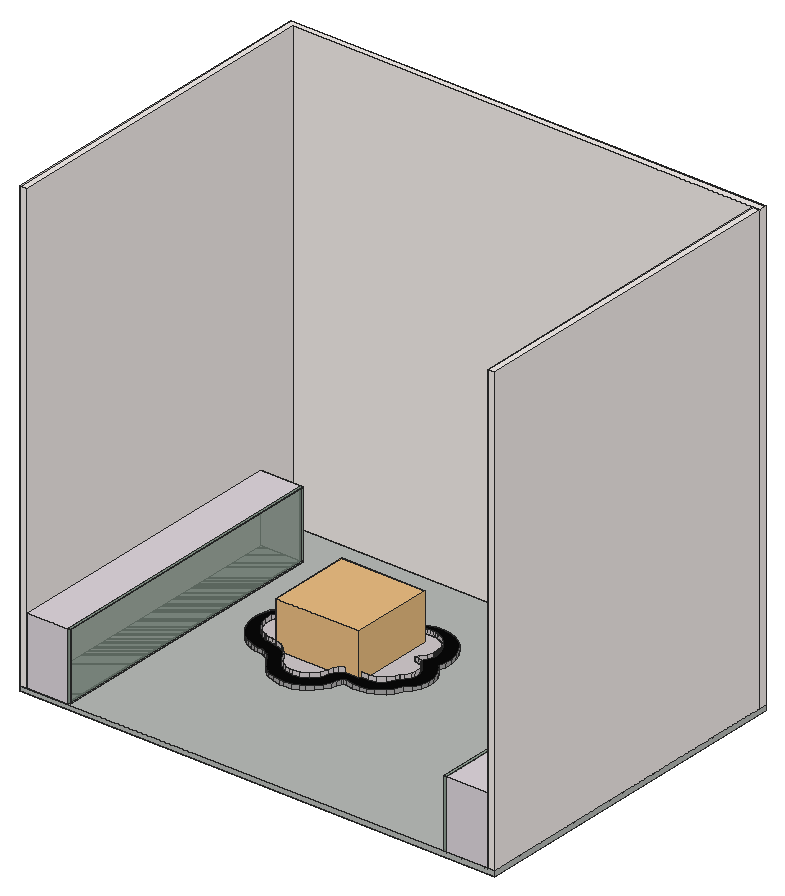
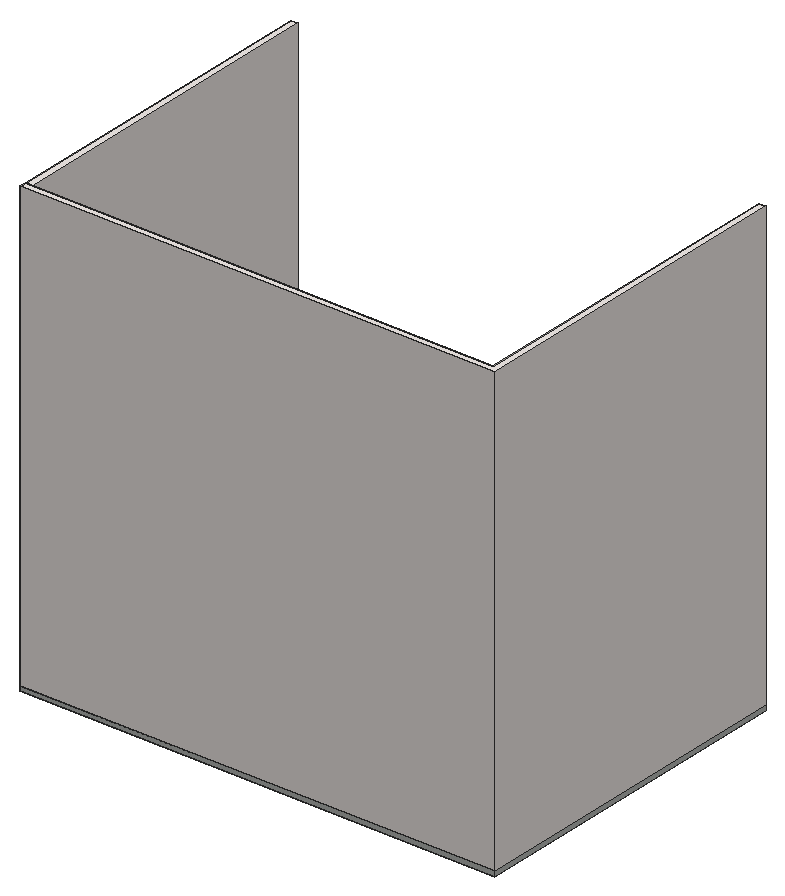
# SketchUp Ruby script. Lengths in inches.
U = 1.inch
M = Sketchup.active_model
def pt(a) = Geom::Point3d.new(a.map { |v| v * U })
def face(e, loops, mat)
  f = e.add_face(loops[0].map { |a| pt(a) })
  loops[1..].each { |l| e.add_face(l.map { |a| pt(a) }).erase! }
  f.material = f.back_material = mat if mat
  f
end
# faces: each face lists its corners as indices into pts; further lists are holes
def faces(e, pts, list, mat = nil) = list.each { |f| face(e, (f[0].is_a?(Array) ? f : [f]).map { |l| l.map { |i| pts[i] } }, mat) }
# xy, xz, yz: faces in a plane at the given z, y or x. An outline is a flat list of corners, or four numbers for a rectangle; further outlines are holes
def ring(l) = l.size == 4 ? [[l[0], l[1]], [l[2], l[1]], [l[2], l[3]], [l[0], l[3]]] : l.each_slice(2).to_a
def flat(e, list, mat, &to3) = list.each { |f| face(e, (f[0].is_a?(Array) ? f : [f]).map { |l| ring(l).map { |u, v| to3.(u, v) } }, mat) }
def xy(e, z, list, mat = nil) = flat(e, list, mat) { |x, y| [x, y, z] }
def xz(e, y, list, mat = nil) = flat(e, list, mat) { |x, z| [x, y, z] }
def yz(e, x, list, mat = nil) = flat(e, list, mat) { |y, z| [x, y, z] }
def lines(e, pts, list) = list.each { |a, b| e.add_line(pt(pts[a]), pt(pts[b])) }
# prism: a flat outline (further loops are holes) pulled along v
def prism(e, loops, v, mat = nil)
  f = face(e, loops, mat); d = Geom::Vector3d.new(v.map { |x| x * U })
  f.pushpull(f.normal.samedirection?(d) ? d.length : -d.length)
end
def box(e, o, s, mat = nil) = prism(e, [[o, [o[0] + s[0], o[1], o[2]], [o[0] + s[0], o[1] + s[1], o[2]], [o[0], o[1] + s[1], o[2]]]], [0, 0, s[2]], mat)
def at(x, y, z, deg = 0) = Geom::Transformation.translation(pt([x, y, z])) * Geom::Transformation.rotation(ORIGIN, Z_AXIS, deg.degrees)
def axes(o, x, y, z) = Geom::Transformation.new([*x, 0, *y, 0, *z, 0, *pt(o).to_a, 1])
def part(name) = M.definitions.add(name)
# library, detail: a bought-in or finely detailed component or shape, given as its bounding box
def library(name, o, s) = part(name).tap { |d| box(d.entities, o, s) }
def detail(e, o, s) = box(e.add_group.entities, o, s)
def put(e, d, t, mat = nil) = e.add_instance(d, t).tap { |i| i.material = mat if mat }
def group(e, t, mat = nil) = e.add_group.tap { |g| g.transformation = t; g.material = mat if mat }.entities
root = M.entities
M.materials.add("0209 AP 9428 SKY PINK").color = [243, 236, 233]
M.materials.add("0265 AP 7147 LAVENDER LAUGH").color = [222, 214, 220]
M.materials.add("Bricks_Tiles_D02_50cm").color = [9, 9, 9]
M.materials.add("Epoch Sky_ Double Herringbone (VR1MIV)").color = [184, 188, 184]
M.materials.add("[Stone_Granite_Midnite]").color = [209, 202, 204]
M.materials.add("[Stone_Vein_Gray]").color = [166, 165, 165]
M.materials.add("[Translucent Glass Corrugated]").color = [141, 158, 145]
M.materials["[Translucent Glass Corrugated]"].alpha = 0.8
c1 = part("Group\#1")
box(c1.entities,[0,0,0],[840,600,8])
c2 = library("Group\#44",[13.4,13.93,0],[164.31,164.31,140.86])
c3 = part("Group41\#1")
p = [[514.8125,1.1875,0],[1.1875,1.1875,0],[1.1875,118.8125,0],[514.8125,118.8125,0]]
lines(c3.entities,p,[[0,1],[1,2],[2,3],[3,0]])
c4 = part("Group42\#1")
xy(c4.entities,2.9375,[[1.1875,1.1875,514.8125,118.8125]])
c5 = part("Group40\#1")
prism(c5.entities,[[[516,120,0],[516,0,0],[0,0,0],[0,120,0]],[[1.1875,118.8125,0],[1.1875,1.1875,0],[514.8125,1.1875,0],[514.8125,118.8125,0]]],[0,0,5.875])
put(c5.entities,c3,at(0,0,0))
put(c5.entities,c4,at(0,0,0))
c6 = part("Group\#11")
xy(c6.entities,0,[[0,72,72,588]])
xy(c6.entities,120,[[0,72,72,588]])
xz(c6.entities,72,[[0,0,72,120]])
xz(c6.entities,588,[[0,0,72,120]])
yz(c6.entities,0,[[72,0,588,120]])
put(c6.entities,c5,axes([72,72,0],[0,1,0],[0,0,1],[1,0,0]),"[Translucent Glass Corrugated]")
xy(root,8,[[286.38,226.11,278.14,226.18,265.97,228.35,254.48,232.88,247.41,237.13,238.03,245.17,230.42,254.91,225.67,263.83,222.52,268.43,218.51,272.29,213.8,275.26,210.37,276.6875,204.93,277.92,198.67,278.46,192.125,279.62,185.71,281.35,177.5,284.68,171.69,287.91,166.19,291.64,162.76,294.44,159.52,297.46,151.1,307.73,146.6875,315.41,142.08,327.86,140.02,340.98,140.12,349.84,142.46,362.91,145.4375,371.25,151.91,382.84,160.55,392.92,168.89,400.18,170.02,404.39,169.07,412.74,168.71,420.7,170.62,441.81,170.86,444.46,171.88,448.31,173.58,454.71,174.94,459.85,181.06,474.55,193.58,493.52,208.59,506.3,231.23,515.95,240.97,517.6,260.68,516.94,265.53,515.95,274.96,513.01,291.39,503.95,296.1,500.41,299.76,497.09,306.35,489.73,313.41,479.34,318.33,474.84,325.77,471.91,332.44,471.86,337.55,473.39,353.76,478.27,366.45,479.05,379.05,477.32,391.06,473.13,402,466.67,411.46,458.18,421.13,444.28,425.8,432.45,428.06,419.94,427.81,407.23,425.05,394.82,432.1,387.375,438.96,375.57,442.49,362.39,442.79,352.14,440.05,338.77,433.89,326.58,424.77,316.43,419.17,306,411.6,296.89,398.99,287.43,388.13,282.72,376.55,280.26,364.72,280.16,350.18,282.69,346.97,281.54,344.64,279.05,342.91,272.72,340.36,264.88,334.63,253.93,326.85,244.34,317.3125,236.47,310.17,232.35,298.59,228.04]],"[Stone_Granite_Midnite]")
xy(root,15.29,[[[286.38,226.11,298.59,228.04,310.17,232.35,317.3125,236.47,326.85,244.34,334.63,253.93,340.36,264.88,342.91,272.72,344.64,279.05,346.97,281.54,350.18,282.69,364.72,280.16,376.55,280.26,388.13,282.72,398.99,287.43,411.6,296.89,419.17,306,424.77,316.43,433.89,326.58,440.05,338.77,442.79,352.14,442.49,362.39,438.96,375.57,432.1,387.375,425.05,394.82,427.81,407.23,428.06,419.94,425.8,432.45,421.13,444.28,411.46,458.18,402,466.67,391.06,473.13,379.05,477.32,366.45,479.05,353.76,478.27,337.55,473.39,332.44,471.86,325.77,471.91,318.33,474.84,313.41,479.34,306.35,489.73,299.76,497.09,296.1,500.41,291.39,503.95,274.96,513.01,265.53,515.95,260.68,516.94,240.97,517.6,231.23,515.95,208.59,506.3,193.58,493.52,181.06,474.55,174.94,459.85,173.58,454.71,171.88,448.31,170.86,444.46,170.62,441.81,168.71,420.7,169.07,412.74,170.02,404.39,168.89,400.18,160.55,392.92,151.91,382.84,145.4375,371.25,142.46,362.91,140.12,349.84,140.02,340.98,142.08,327.86,146.6875,315.41,151.1,307.73,159.52,297.46,162.76,294.44,166.19,291.64,171.69,287.91,177.5,284.68,185.71,281.35,192.125,279.62,198.67,278.46,204.93,277.92,210.37,276.6875,213.8,275.26,218.51,272.29,222.52,268.43,225.67,263.83,230.42,254.91,238.03,245.17,247.41,237.13,254.48,232.88,265.97,228.35,278.14,226.18],[283.33,249.2,277.3125,249.46,269.78,251.32,262.77,254.64,256.55,259.29,249.93,267.22,244.19,277.79,235.37,288.23,224.0625,295.92,211.11,300.28,204.3,301.11,198.55,301.8,195.08,302.62,192.9375,303.25,190.8,304.2,190.22,304.25,185,306.78,175.8,313.79,167.41,325.53,163.75,336.51,163.43,350.94,167.83,364.6875,176.48,376.24,186.71,385.52,190.37,391.69,192.09,396.23,193.05,402.18,192.56,412.99,191.92,427.37,193.5,440.07,196.78,452.45,201.7,464.27,208.5625,475.52,218.26,484.97,230.125,491.51,243.29,494.66,256.83,494.2,269.76,490.17,272.78,488.64,277.1,485.93,281.15,482.86,290.2,472.77,299.07,460.86,310.82,452.68,321.75,449.2,336.07,449.08,338.89,449.63,343.04,450.82,347.06,452.38,352.13,454.28,356.08,455.24,361.45,455.94,365.51,456.01,370.9,455.46,372.22,455.19,373.55,454.92,376.17,454.21,388.23,448.17,397.7,438.5625,401.69,431.49,403.55,426.41,404.22,423.78,404.72,421.12,404.85,418.74,404.875,418.25,405.01,415.75,405.11,413.92,405.16,413.01,405.01,411.67,404.78,409.65,402.35,399.82,395.43,388.24,391.67,384.34,397.375,383.69,404.5625,381.0625,406.49,379.59,408,378.45,411.39,375.86,411.5,375.7,411.92,375.15,412.05,374.99,416.58,369.03,417.85,365.55,419.2,361.84,419.35,350.41,417.72,344.9,412.68,336.8,408.45,332.9,405.24,330.8,403.8,326.12,397.57,315.62,386.02,306.66,374.31,303.22,362.12,303.88,361.75,303.98,361.46,304.05,361.3125,304.09,357.77,305.03,349.66,305.77,343.61,304.89,336.05,301.87,326.86,293.88,323.65,288.67,321.12,280.93,316.71,268.8125,306.59,257.15,295.21,251.08]]],"Bricks_Tiles_D02_50cm")
p = [[278.14,226.18,8],[286.38,226.11,8],[286.38,226.11,15.29],[278.14,226.18,15.29],[298.59,228.04,8],[298.59,228.04,15.29],
  [265.97,228.35,8],[265.97,228.35,15.29],[310.17,232.35,8],[310.17,232.35,15.29],[254.48,232.88,8],[254.48,232.88,15.29],
  [317.3125,236.47,8],[317.3125,236.47,15.29],[247.41,237.13,8],[247.41,237.13,15.29],[326.85,244.34,8],[326.85,244.34,15.29],
  [238.03,245.17,8],[238.03,245.17,15.29],[334.63,253.93,8],[334.63,253.93,15.29],[230.42,254.91,8],[230.42,254.91,15.29],
  [340.36,264.88,8],[340.36,264.88,15.29],[225.67,263.83,8],[225.67,263.83,15.29],[222.52,268.43,8],[222.52,268.43,15.29],
  [342.91,272.72,8],[342.91,272.72,15.29],[218.51,272.29,8],[218.51,272.29,15.29],[213.8,275.26,8],[213.8,275.26,15.29],
  [344.64,279.05,8],[344.64,279.05,15.29],[210.37,276.6875,8],[210.37,276.6875,15.29],[204.93,277.92,8],[204.93,277.92,15.29],
  [198.67,278.46,8],[198.67,278.46,15.29],[192.125,279.62,8],[192.125,279.62,15.29],[346.97,281.54,8],[346.97,281.54,15.29],
  [185.71,281.35,8],[185.71,281.35,15.29],[350.18,282.69,8],[364.72,280.16,8],[364.72,280.16,15.29],[350.18,282.69,15.29],
  [376.55,280.26,8],[376.55,280.26,15.29],[388.13,282.72,8],[388.13,282.72,15.29],[177.5,284.68,8],[177.5,284.68,15.29],
  [398.99,287.43,8],[398.99,287.43,15.29],[171.69,287.91,8],[171.69,287.91,15.29],[411.6,296.89,8],[411.6,296.89,15.29],
  [166.19,291.64,8],[166.19,291.64,15.29],[162.76,294.44,8],[162.76,294.44,15.29],[161.14,295.95,8],[161.14,295.95,15.29],
  [159.52,297.46,8],[159.52,297.46,15.29],[419.17,306,8],[419.17,306,15.29],[151.1,307.73,8],[151.1,307.73,15.29],
  [424.77,316.43,8],[424.77,316.43,15.29],[146.6875,315.41,8],[146.6875,315.41,15.29],[142.08,327.86,8],[142.08,327.86,15.29],
  [433.89,326.58,8],[433.89,326.58,15.29],[440.05,338.77,8],[440.05,338.77,15.29],[140.02,340.98,8],[140.02,340.98,15.29],
  [442.79,352.14,8],[442.79,352.14,15.29],[140.12,349.84,8],[140.12,349.84,15.29],[142.46,362.91,8],[142.46,362.91,15.29],
  [442.49,362.39,8],[442.49,362.39,15.29],[438.96,375.57,8],[438.96,375.57,15.29],[145.4375,371.25,8],[145.4375,371.25,15.29],
  [151.91,382.84,8],[151.91,382.84,15.29],[432.1,387.375,8],[432.1,387.375,15.29],[160.55,392.92,8],[160.55,392.92,15.29],
  [425.05,394.82,8],[425.05,394.82,15.29],[168.89,400.18,8],[168.89,400.18,15.29],[427.81,407.23,8],[427.81,407.23,15.29],
  [170.02,404.39,8],[170.02,404.39,15.29],[169.07,412.74,8],[169.07,412.74,15.29],[428.06,419.94,8],[428.06,419.94,15.29],
  [168.71,420.7,8],[168.71,420.7,15.29],[425.8,432.45,8],[425.8,432.45,15.29],[170.62,441.81,8],[170.62,441.81,15.29],
  [421.13,444.28,8],[421.13,444.28,15.29],[170.86,444.46,8],[170.86,444.46,15.29],[411.46,458.18,8],[411.46,458.18,15.29],
  [171.88,448.31,8],[171.88,448.31,15.29],[173.58,454.71,8],[173.58,454.71,15.29],[174.94,459.85,8],[174.94,459.85,15.29],
  [402,466.67,8],[402,466.67,15.29],[181.06,474.55,8],[181.06,474.55,15.29],[391.06,473.13,8],[391.06,473.13,15.29],
  [325.77,471.91,8],[318.33,474.84,8],[318.33,474.84,15.29],[325.77,471.91,15.29],[332.44,471.86,8],[332.44,471.86,15.29],
  [337.55,473.39,8],[337.55,473.39,15.29],[379.05,477.32,8],[379.05,477.32,15.29],[353.76,478.27,8],[353.76,478.27,15.29],
  [193.58,493.52,8],[193.58,493.52,15.29],[313.41,479.34,8],[313.41,479.34,15.29],[366.45,479.05,8],[366.45,479.05,15.29],
  [306.35,489.73,8],[306.35,489.73,15.29],[299.76,497.09,8],[299.76,497.09,15.29],[208.59,506.3,8],[208.59,506.3,15.29],
  [296.1,500.41,8],[296.1,500.41,15.29],[291.39,503.95,8],[291.39,503.95,15.29],[274.96,513.01,8],[274.96,513.01,15.29],
  [231.23,515.95,8],[231.23,515.95,15.29],[265.53,515.95,8],[265.53,515.95,15.29],[240.97,517.6,8],[240.97,517.6,15.29],
  [260.68,516.94,8],[260.68,516.94,15.29],[277.3125,249.46,22.57],[277.3125,249.46,15.29],[283.33,249.2,15.29],[283.33,249.2,22.57],
  [295.21,251.08,15.29],[295.21,251.08,22.57],[269.78,251.32,22.57],[269.78,251.32,15.29],[306.59,257.15,15.29],[306.59,257.15,22.57],
  [262.77,254.64,22.57],[262.77,254.64,15.29],[256.55,259.29,22.57],[256.55,259.29,15.29],[316.71,268.8125,15.29],[316.71,268.8125,22.57],
  [249.93,267.22,22.57],[249.93,267.22,15.29],[244.19,277.79,22.57],[244.19,277.79,15.29],[321.12,280.93,15.29],[321.12,280.93,22.57],
  [235.37,288.23,22.57],[235.37,288.23,15.29],[323.65,288.67,15.29],[323.65,288.67,22.57],[224.0625,295.92,22.57],[224.0625,295.92,15.29],
  [326.86,293.88,15.29],[326.86,293.88,22.57],[336.05,301.87,15.29],[336.05,301.87,22.57],[211.11,300.28,22.57],[211.11,300.28,15.29],
  [204.3,301.11,22.57],[204.3,301.11,15.29],[198.55,301.8,22.57],[198.55,301.8,15.29],[195.08,302.62,22.57],[195.08,302.62,15.29],
  [343.61,304.89,15.29],[343.61,304.89,22.57],[192.9375,303.25,22.57],[192.9375,303.25,15.29],[190.8,304.2,22.57],[190.8,304.2,15.29],
  [362.12,303.88,22.57],[362.12,303.88,15.29],[374.31,303.22,15.29],[374.31,303.22,22.57],[386.02,306.66,15.29],[386.02,306.66,22.57],
  [361.75,303.98,22.57],[361.75,303.98,15.29],[361.46,304.05,22.57],[361.46,304.05,15.29],[357.77,305.03,22.57],[357.77,305.03,15.29],
  [361.3125,304.09,15.29],[361.3125,304.09,22.57],[190.22,304.25,22.57],[185,306.78,22.57],[185,306.78,15.29],[190.22,304.25,15.29],
  [349.66,305.77,15.29],[349.66,305.77,22.57],[397.57,315.62,15.29],[397.57,315.62,22.57],[175.8,313.79,22.57],[175.8,313.79,15.29],
  [167.41,325.53,22.57],[167.41,325.53,15.29],[403.8,326.12,15.29],[403.8,326.12,22.57],[163.75,336.51,22.57],[163.75,336.51,15.29],
  [405.24,330.8,15.29],[405.24,330.8,22.57],[408.45,332.9,15.29],[408.45,332.9,22.57],[412.68,336.8,15.29],[412.68,336.8,22.57],
  [163.43,350.94,22.57],[163.43,350.94,15.29],[417.72,344.9,15.29],[417.72,344.9,22.57],[419.35,350.41,15.29],[419.35,350.41,22.57],
  [419.2,361.84,15.29],[419.2,361.84,22.57],[167.83,364.6875,22.57],[167.83,364.6875,15.29],[417.85,365.55,15.29],[417.85,365.55,22.57],
  [176.48,376.24,22.57],[176.48,376.24,15.29],[416.58,369.03,15.29],[416.58,369.03,22.57],[412.05,374.99,15.29],[412.05,374.99,22.57],
  [411.92,375.15,15.29],[411.92,375.15,22.57],[411.5,375.7,15.29],[411.5,375.7,22.57],[411.39,375.86,15.29],[411.39,375.86,22.57],
  [408,378.45,15.29],[408,378.45,22.57],[186.71,385.52,22.57],[186.71,385.52,15.29],[406.49,379.59,15.29],[406.49,379.59,22.57],
  [404.5625,381.0625,15.29],[404.5625,381.0625,22.57],[397.375,383.69,15.29],[397.375,383.69,22.57],[391.67,384.34,15.29],[391.67,384.34,22.57],
  [395.43,388.24,15.29],[395.43,388.24,22.57],[190.37,391.69,22.57],[190.37,391.69,15.29],[402.35,399.82,15.29],[402.35,399.82,22.57],
  [192.09,396.23,22.57],[192.09,396.23,15.29],[193.05,402.18,22.57],[193.05,402.18,15.29],[404.78,409.65,15.29],[404.78,409.65,22.57],
  [192.56,412.99,22.57],[192.56,412.99,15.29],[405.01,411.67,15.29],[405.01,411.67,22.57],[405.16,413.01,15.29],[405.16,413.01,22.57],
  [191.92,427.37,22.57],[191.92,427.37,15.29],[405.11,413.92,15.29],[405.11,413.92,22.57],[405.01,415.75,15.29],[405.01,415.75,22.57],
  [404.875,418.25,15.29],[404.875,418.25,22.57],[404.85,418.74,15.29],[404.85,418.74,22.57],[404.72,421.12,15.29],[404.72,421.12,22.57],
  [404.22,423.78,22.57],[404.22,423.78,15.29],[403.55,426.41,22.57],[403.55,426.41,15.29],[401.69,431.49,22.57],[401.69,431.49,15.29],
  [193.5,440.07,22.57],[193.5,440.07,15.29],[397.7,438.5625,15.29],[397.7,438.5625,22.57],[388.23,448.17,15.29],[388.23,448.17,22.57],
  [196.78,452.45,22.57],[196.78,452.45,15.29],[376.17,454.21,15.29],[376.17,454.21,22.57],[336.07,449.08,22.57],[336.07,449.08,15.29],
  [321.75,449.2,15.29],[321.75,449.2,22.57],[338.89,449.63,22.57],[338.89,449.63,15.29],[310.82,452.68,15.29],[310.82,452.68,22.57],
  [343.04,450.82,22.57],[343.04,450.82,15.29],[347.06,452.38,22.57],[347.06,452.38,15.29],[201.7,464.27,22.57],[201.7,464.27,15.29],
  [352.13,454.28,22.57],[352.13,454.28,15.29],[299.07,460.86,15.29],[299.07,460.86,22.57],[373.55,454.92,15.29],[373.55,454.92,22.57],
  [356.08,455.24,22.57],[356.08,455.24,15.29],[372.22,455.19,15.29],[372.22,455.19,22.57],[361.45,455.94,22.57],[361.45,455.94,15.29],
  [370.9,455.46,15.29],[370.9,455.46,22.57],[365.51,456.01,15.29],[365.51,456.01,22.57],[290.2,472.77,15.29],[290.2,472.77,22.57],
  [208.5625,475.52,22.57],[208.5625,475.52,15.29],[281.15,482.86,15.29],[281.15,482.86,22.57],[218.26,484.97,22.57],[218.26,484.97,15.29],
  [277.1,485.93,15.29],[277.1,485.93,22.57],[230.125,491.51,22.57],[230.125,491.51,15.29],[272.78,488.64,15.29],[272.78,488.64,22.57],
  [269.76,490.17,15.29],[269.76,490.17,22.57],[256.83,494.2,15.29],[256.83,494.2,22.57],[243.29,494.66,22.57],[243.29,494.66,15.29],
  [292.23,503.49,8]]
faces(root,p,[[0,1,2,3],[1,4,5,2],[6,0,3,7],[4,8,9,5],[10,6,7,11],[8,12,13,9],[14,10,11,15],[12,16,17,13],
  [18,14,15,19],[16,20,21,17],[22,18,19,23],[20,24,25,21],[26,22,23,27],[28,26,27,29],[24,30,31,25],[32,28,29,33],
  [34,32,33,35],[30,36,37,31],[38,34,35,39],[40,38,39,41],[42,40,41,43],[44,42,43,45],[36,46,47,37],[48,44,45,49],
  [50,51,52,53],[51,54,55,52],[54,56,57,55],[58,48,49,59],[46,50,53,47],[56,60,61,57],[62,58,59,63],[60,64,65,61],
  [66,62,63,67],[68,66,67,69],[70,68,69,71],[72,70,71,73],[64,74,75,65],[76,72,73,77],[74,78,79,75],[80,76,77,81],
  [82,80,81,83],[78,84,85,79],[84,86,87,85],[88,82,83,89],[86,90,91,87],[92,88,89,93],[94,92,93,95],[90,96,97,91],
  [96,98,99,97],[100,94,95,101],[102,100,101,103],[98,104,105,99],[106,102,103,107],[104,108,109,105],[110,106,107,111],[108,112,113,109],
  [114,110,111,115],[116,114,115,117],[112,118,119,113],[120,116,117,121],[118,122,123,119],[124,120,121,125],[122,126,127,123],[128,124,125,129],
  [126,130,131,127],[132,128,129,133],[134,132,133,135],[136,134,135,137],[130,138,139,131],[140,136,137,141],[138,142,143,139],[144,145,146,147],
  [148,144,147,149],[150,148,149,151],[142,152,153,143],[154,150,151,155],[156,140,141,157],[145,158,159,146],[152,160,161,153],[160,154,155,161],
  [158,162,163,159],[162,164,165,163],[166,156,157,167],[164,168,169,165],[168,170,171,169],[170,172,173,171],[174,166,167,175],[172,176,177,173],
  [178,174,175,179],[176,180,181,177],[180,178,179,181]],"[Stone_Vein_Gray]")
faces(root,p,[[182,183,184,185],[185,184,186,187],[188,189,183,182],[187,186,190,191],[192,193,189,188],[194,195,193,192],[191,190,196,197],[198,199,195,194],
  [200,201,199,198],[197,196,202,203],[204,205,201,200],[203,202,206,207],[208,209,205,204],[207,206,210,211],[211,210,212,213],[214,215,209,208],
  [216,217,215,214],[218,219,217,216],[220,221,219,218],[213,212,222,223],[224,225,221,220],[224,226,227,225],[228,229,230,231],[231,230,232,233],
  [234,235,229,228],[236,237,235,234],[238,239,240,241],[241,240,237,236],[242,243,244,245],[226,242,245,227],[223,222,246,247],[247,246,239,238],
  [233,232,248,249],[250,251,244,243],[252,253,251,250],[249,248,254,255],[256,257,253,252],[255,254,258,259],[259,258,260,261],[261,260,262,263],
  [264,265,257,256],[263,262,266,267],[267,266,268,269],[269,268,270,271],[272,273,265,264],[271,270,274,275],[276,277,273,272],[275,274,278,279],
  [279,278,280,281],[281,280,282,283],[283,282,284,285],[285,284,286,287],[287,286,288,289],[290,291,277,276],[289,288,292,293],[293,292,294,295],
  [295,294,296,297],[297,296,298,299],[299,298,300,301],[302,303,291,290],[301,300,304,305],[306,307,303,302],[308,309,307,306],[305,304,310,311],
  [312,313,309,308],[311,310,314,315],[315,314,316,317],[318,319,313,312],[317,316,320,321],[321,320,322,323],[323,322,324,325],[325,324,326,327],
  [327,326,328,329],[334,332,333,335],[336,337,319,318],[334,335,338,339],[339,338,340,341],[342,343,337,336],[341,340,344,345],[346,347,348,349],
  [350,351,347,346],[349,348,352,353],[354,355,351,350],[356,357,355,354],[358,359,343,342],[360,361,357,356],[353,352,362,363],[345,344,364,365],
  [366,367,361,360],[365,364,368,369],[370,371,367,366],[369,368,372,373],[373,372,374,375],[375,374,371,370],[363,362,376,377],[378,379,359,358],
  [377,376,380,381],[382,383,379,378],[381,380,384,385],[386,387,383,382],[385,384,388,389],[389,388,390,391],[391,390,392,393],[394,395,387,386],
  [393,392,395,394]],"[Stone_Granite_Midnite]")
faces(root,p,[[330,329,328,331],[332,330,331,333]],"Bricks_Tiles_D02_50cm")
lines(root,p,[[170,396]])
put(root,c1,at(0,0,0),"Epoch Sky_ Double Herringbone (VR1MIV)")
put(root,c2,axes([200.48,287.83,3.42],[0.89562,0,0],[0,0.88603,0],[0,0,0.6072]),"[Stone_Granite_Midnite]")
put(root,c6,at(12,-72,8),"0265 AP 7147 LAVENDER LAUGH")
g1 = group(root,at(0,0,8),"0209 AP 9428 SKY PINK")
prism(g1,[[[12,588,0],[12,0,0],[0,0,0],[0,600,0],[840,600,0],[840,588,0]]],[0,0,792])
g2 = group(root,at(828,0,8),"0209 AP 9428 SKY PINK")
box(g2,[0,0,0],[12,588,792])
put(root,c6,axes([828,-72,8],[-1,0,0],[0,1,0],[0,0,1]),"0265 AP 7147 LAVENDER LAUGH")
